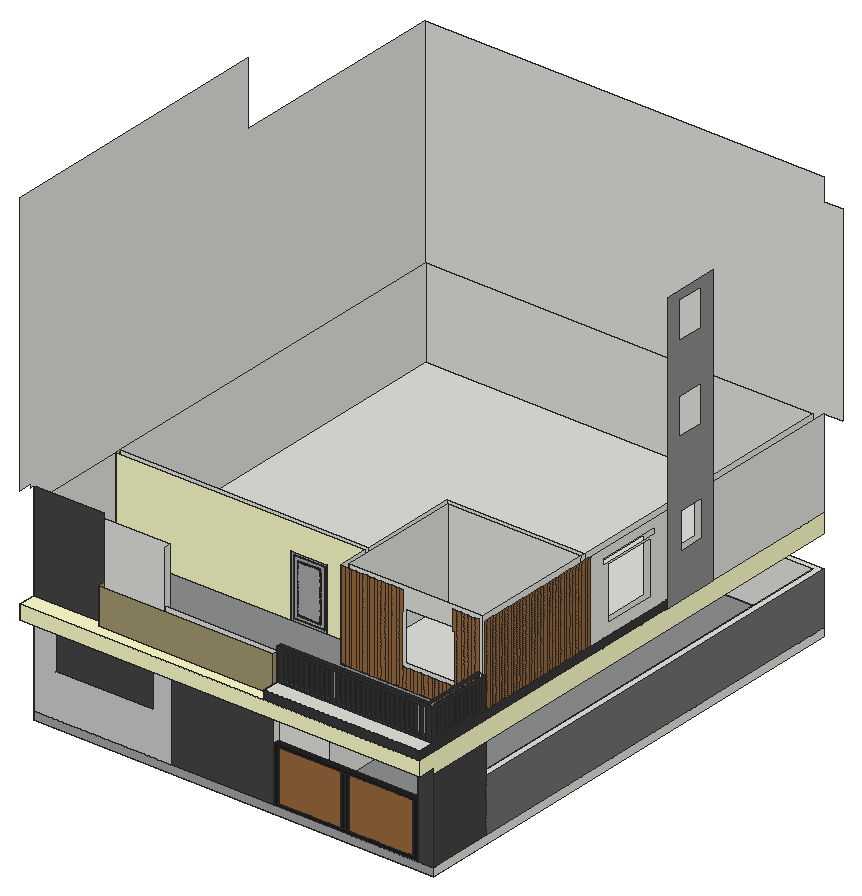
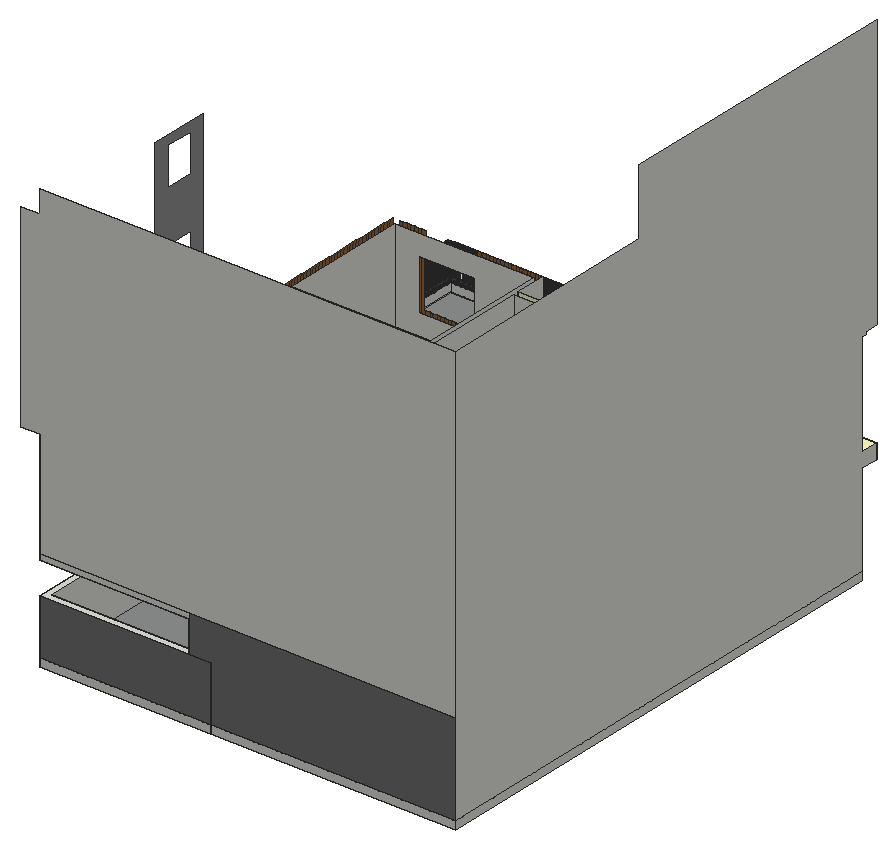
# SketchUp Ruby script. Lengths in inches.
U = 1.inch
M = Sketchup.active_model
def pt(a) = Geom::Point3d.new(a.map { |v| v * U })
def face(e, loops, mat)
  f = e.add_face(loops[0].map { |a| pt(a) })
  loops[1..].each { |l| e.add_face(l.map { |a| pt(a) }).erase! }
  f.material = f.back_material = mat if mat
  f
end
# faces: each face lists its corners as indices into pts; further lists are holes
def faces(e, pts, list, mat = nil) = list.each { |f| face(e, (f[0].is_a?(Array) ? f : [f]).map { |l| l.map { |i| pts[i] } }, mat) }
# xy, xz, yz: faces in a plane at the given z, y or x. An outline is a flat list of corners, or four numbers for a rectangle; further outlines are holes
def ring(l) = l.size == 4 ? [[l[0], l[1]], [l[2], l[1]], [l[2], l[3]], [l[0], l[3]]] : l.each_slice(2).to_a
def flat(e, list, mat, &to3) = list.each { |f| face(e, (f[0].is_a?(Array) ? f : [f]).map { |l| ring(l).map { |u, v| to3.(u, v) } }, mat) }
def xy(e, z, list, mat = nil) = flat(e, list, mat) { |x, y| [x, y, z] }
def xz(e, y, list, mat = nil) = flat(e, list, mat) { |x, z| [x, y, z] }
def yz(e, x, list, mat = nil) = flat(e, list, mat) { |y, z| [x, y, z] }
def lines(e, pts, list) = list.each { |a, b| e.add_line(pt(pts[a]), pt(pts[b])) }
# prism: a flat outline (further loops are holes) pulled along v
def prism(e, loops, v, mat = nil)
  f = face(e, loops, mat); d = Geom::Vector3d.new(v.map { |x| x * U })
  f.pushpull(f.normal.samedirection?(d) ? d.length : -d.length)
end
def box(e, o, s, mat = nil) = prism(e, [[o, [o[0] + s[0], o[1], o[2]], [o[0] + s[0], o[1] + s[1], o[2]], [o[0], o[1] + s[1], o[2]]]], [0, 0, s[2]], mat)
def at(x, y, z, deg = 0) = Geom::Transformation.translation(pt([x, y, z])) * Geom::Transformation.rotation(ORIGIN, Z_AXIS, deg.degrees)
def axes(o, x, y, z) = Geom::Transformation.new([*x, 0, *y, 0, *z, 0, *pt(o).to_a, 1])
def part(name) = M.definitions.add(name)
# library, detail: a bought-in or finely detailed component or shape, given as its bounding box
def library(name, o, s) = part(name).tap { |d| box(d.entities, o, s) }
def detail(e, o, s) = box(e.add_group.entities, o, s)
def put(e, d, t, mat = nil) = e.add_instance(d, t).tap { |i| i.material = mat if mat }
def group(e, t, mat = nil) = e.add_group.tap { |g| g.transformation = t; g.material = mat if mat }.entities
root = M.entities
M.materials.add("[Blacktop Old 02]").color = [143, 145, 145]
M.materials.add("[Carrera Marble]").color = [207, 207, 207]
M.materials.add("[Color A08]1").color = [91, 11, 0]
M.materials.add("[Color E01]").color = [255, 255, 204]
M.materials.add("[Color M03]").color = [170, 170, 170]
M.materials.add("[Color M04]").color = [142, 142, 142]
M.materials.add("[Color M05]").color = [114, 114, 114]
M.materials.add("[Color M07]").color = [58, 58, 58]
M.materials.add("[Color M08]").color = [30, 30, 30]
M.materials.add("[Granite Dark Gray]1").color = [69, 68, 68]
M.materials.add("[Granite Dark Gray]2").color = [69, 68, 68]
M.materials.add("[Stone Vein Gray]").color = [166, 165, 165]
M.materials.add("[Wood Floor]").color = [155, 105, 61]
M.materials.add("[Wood Lumber ButtJoined]").color = [164, 152, 112]
c1 = part("Group\#3")
xy(c1.entities,0,[[0,0,48,5]],"[Color M03]")
xy(c1.entities,2.98,[[2.98,0,45.02,5]],"[Color M03]")
xy(c1.entities,81.02,[[2.98,0,45.02,5]],"[Color M03]")
xy(c1.entities,84,[[0,0,48,5]],"[Color M03]")
xz(c1.entities,0,[[[2.98,2.98,45.02,81.02],[4.42,4.42,43.58,79.58]],[[8.55,8.55,39.45,75.45],[9.61,9.61,38.39,74.39]]],"[Color A08]1")
xz(c1.entities,0,[[[0,0,48,84],[2.98,2.98,45.02,81.02]],[[4.42,4.42,43.58,79.58],[8.55,8.55,39.45,75.45]],[9.61,9.61,38.39,74.39]],"[Color M03]")
xz(c1.entities,5,[[[0,0,48,84],[2.98,2.98,45.02,81.02]]],"[Color M03]")
yz(c1.entities,0,[[0,0,5,84]],"[Color M03]")
yz(c1.entities,2.98,[[0,2.98,5,81.02]],"[Color M03]")
yz(c1.entities,45.02,[[0,2.98,5,81.02]],"[Color M03]")
yz(c1.entities,48,[[0,0,5,84]],"[Color M03]")
xy(root,-10.6875,[[0,27,540,687]])
xy(root,0,[[[0,27,324.55,27,324.55,36,9,36,9,94.1875,345.75,94.1875,345.75,678,317.875,678,317.875,687,0,687],[9,100.1875,311.3125,678]],[324.55,27,518.875,36],[518.875,27,540,114.78],[9,100.1875,311.3125,678],[531,114.78,540,114.78,540,687,317.875,687,317.875,678,531,678]])
xy(root,0,[[9,36,518.875,36,518.875,114.78,531,114.78,531,678,345.75,678,345.75,94.1875,9,94.1875]],"[Blacktop Old 02]")
xy(root,72,[[531,114.78,540,114.78,540,687,345.75,687,345.75,678,531,678],[317.875,678,345.75,687]])
xy(root,102.125,[[9,100.1875,311.3125,678]])
xy(root,113.5625,[[324.55,27,324.55,94.1875,345.75,94.1875,345.75,687,531,687,531,114.78,518.875,114.78,518.875,27],[518.875,27,531,36],[518.875,36,531,114.78],[531,114.78,540,687]])
xy(root,116.6875,[[9,36,324.55,94.1875]])
xy(root,120,[[0,3.875,324.55,27],[324.55,3.875,531,27],[531,3.875,540,27]])
xy(root,139.5625,[[330.17,3.875,540,27],[176.76,27,176.76,31.22,531,31.22,531,113.4375,540,113.4375,540,27],[351.1875,121.0625,531,288],[9,161.0625,345.1875,161.0625,345.1875,294,531,294,531,678,9,678]])
xy(root,139.5625,[[0,3.875,330.17,3.875,330.17,18,94.8,18,94.8,27,0,27]],"[Color E01]")
xy(root,140.19,[[176.76,31.22,531,31.22,531,113.4375,345.1875,113.4375,345.1875,154.125,294.2,154.125,294.2,161.0625,246.2,161.0625,246.2,154.125,9,154.125,9,36,176.76,36]],"[Blacktop Old 02]")
xy(root,151.5625,[[330.17,3.875,540,24.875],[330.17,24.875,330.17,31.22,531,31.22,531,113.4375,540,113.4375,540,24.875],[176.76,27,330.17,31.22]])
xy(root,154.78,[[337.98,26.53,339.42,29.97],[344.98,26.53,346.42,29.97],[488.48,26.53,489.92,29.97],[494.98,26.53,496.42,29.97],[501.48,26.53,502.92,29.97],
  [507.98,26.53,509.42,29.97],[514.3,26.53,515.73,29.97],[522.48,26.53,523.92,29.97]])
xy(root,154.78,[[[333.39,24.875,531,31.22],[337.98,26.53,339.42,29.97],[344.98,26.53,346.42,29.97],[351.98,26.53,353.42,29.97],[358.98,26.53,360.42,29.97],[365.98,26.53,367.42,29.97],[372.98,26.53,374.42,29.97],[379.98,26.53,381.42,29.97],[386.98,26.53,388.42,29.97],[393.98,26.53,395.42,29.97],[400.98,26.53,402.42,29.97],[407.98,26.53,409.42,29.97],[414.98,26.53,416.42,29.97],[421.98,26.53,423.42,29.97],[428.98,26.53,430.42,29.97],[435.98,26.53,437.42,29.97],[442.98,26.53,444.42,29.97],[449.48,26.53,450.92,29.97],[455.98,26.53,457.42,29.97],[462.48,26.53,463.92,29.97],[468.98,26.53,470.42,29.97],[475.48,26.53,476.92,29.97],[481.98,26.53,483.42,29.97],[488.48,26.53,489.92,29.97],[494.98,26.53,496.42,29.97],[501.48,26.53,502.92,29.97],[507.98,26.53,509.42,29.97],[514.3,26.53,515.73,29.97],[522.48,26.53,523.92,29.97]]],"[Color M07]")
xy(root,155.78,[[533.85,35.98,537.54,37.92],[533.85,42.8,537.54,44.73],[533.85,49.61,537.54,51.55],[533.85,56.42,537.54,58.36],[533.85,63.23,537.54,65.17],
  [533.85,70.05,537.54,71.98],[533.85,76.86,537.54,78.8],[533.85,83.67,537.54,85.61],[533.85,90.48,537.54,92.42],[533.85,97.3,537.54,99.23],
  [533.85,104.11,537.54,106.05]])
xy(root,155.78,[[[531,31.22,540,109.22],[533.85,35.98,537.54,37.92],[533.85,42.8,537.54,44.73],[533.85,49.61,537.54,51.55],[533.85,56.42,537.54,58.36],[533.85,63.23,537.54,65.17],[533.85,70.05,537.54,71.98],[533.85,76.86,537.54,78.8],[533.85,83.67,537.54,85.61],[533.85,90.48,537.54,92.42],[533.85,97.3,537.54,99.23],[533.85,104.11,537.54,106.05]]],"[Color M07]")
xz(root,3.875,[[0,120,540,139.5625]],"[Color E01]")
xz(root,3.875,[[330.17,139.5625,540,151.5625]],"[Color M07]")
xz(root,18,[[94.8,139.5625,330.17,188.5625]],"[Wood Lumber ButtJoined]")
xz(root,24.875,[[330.17,151.5625,531,151.5625,531,154.78,333.39,154.78,333.39,192.35,531,192.35,531,195.5625,330.17,195.5625],[531,151.5625,540,195.5625]],"[Color M07]")
xz(root,26.53,[[337.98,154.78,339.42,192.35],[344.98,154.78,346.42,192.09],[351.98,154.78,353.42,192.4],[358.98,154.78,360.42,192.35],[365.98,154.78,367.42,192.34],
  [372.98,154.78,374.42,192.28],[379.98,154.78,381.42,192.65],[386.98,154.78,388.42,193.16],[393.98,154.78,395.42,192.35],[400.98,154.78,402.42,192.35],
  [407.98,154.78,409.42,192.35],[414.98,154.78,416.42,193.4],[421.98,154.78,423.42,193.03],[428.98,154.78,430.42,192.35],[435.98,154.78,437.42,192.4],
  [442.98,154.78,444.42,193.47],[449.48,154.78,450.92,192.35],[455.98,154.78,457.42,192.28],[462.48,154.78,463.92,194.84],[468.98,154.78,470.42,192.34],
  [475.48,154.78,476.92,192.35],[481.98,154.78,483.42,192.34],[488.48,154.78,489.92,192.35],[494.98,154.78,496.42,192.35],[501.48,154.78,502.92,192.34],
  [507.98,154.78,509.42,192.35],[514.3,154.78,515.73,192.35],[522.48,154.78,523.92,195.5625]],"[Color M07]")
xz(root,27,[[176.76,139.5625,330.17,151.5625],[176.76,151.5625,330.17,188.5625]])
xz(root,27,[[[0,0,184.8,120],[29.8,57.58,161.98,104.58]]],"[Carrera Marble]")
xz(root,27,[[184.8,0,324.55,0,324.55,113.5625,531,113.5625,531,120,184.8,120],[0,139.5625,94.8,272.3125]],"[Granite Dark Gray]1")
xz(root,27,[[518.875,0,540,0,540,120,531,120,531,113.5625,518.875,113.5625],[29.8,57.58,161.98,104.58]],"[Granite Dark Gray]2")
xz(root,27,[[0,-10.6875,540,0]],"[Stone Vein Gray]")
xz(root,29.97,[[337.98,154.78,339.42,192.35],[344.98,154.78,346.42,192.09],[351.98,154.78,353.42,192.4],[358.98,154.78,360.42,192.35],[365.98,154.78,367.42,192.34],
  [372.98,154.78,374.42,192.28],[379.98,154.78,381.42,192.65],[386.98,154.78,388.42,193.16],[393.98,154.78,395.42,192.35],[400.98,154.78,402.42,192.35],
  [407.98,154.78,409.42,192.35],[414.98,154.78,416.42,193.4],[421.98,154.78,423.42,193.03],[428.98,154.78,430.42,192.35],[435.98,154.78,437.42,192.4],
  [442.98,154.78,444.42,193.47],[449.48,154.78,450.92,192.35],[455.98,154.78,457.42,192.28],[462.48,154.78,463.92,194.84],[468.98,154.78,470.42,192.34],
  [475.48,154.78,476.92,192.35],[481.98,154.78,483.42,192.34],[488.48,154.78,489.92,192.35],[494.98,154.78,496.42,192.35],[501.48,154.78,502.92,192.34],
  [507.98,154.78,509.42,192.35],[514.3,154.78,515.73,192.35],[522.48,154.78,523.92,195.5625]],"[Color M07]")
xz(root,31.22,[[176.76,139.5625,531,140.19],[176.76,140.19,531,151.5625]])
xz(root,31.22,[[330.17,151.5625,330.17,195.5625,531,195.5625,531,192.35,333.39,192.35,333.39,154.78,531,154.78,531,151.5625],[531,155.78,540,191.35]],"[Color M07]")
xz(root,35.98,[[533.85,155.78,537.54,191.28]],"[Color M07]")
xz(root,36,[[9,0,324.55,116.6875],[9,139.5625,176.76,140.19],[9,140.19,176.76,259.5625]])
xz(root,37.92,[[533.85,155.78,537.54,191.28]],"[Color M07]")
xz(root,42.8,[[533.85,155.78,537.54,191.4]],"[Color M07]")
xz(root,44.73,[[533.85,155.78,537.54,191.4]],"[Color M07]")
xz(root,49.61,[[533.85,155.78,537.54,191.34]],"[Color M07]")
xz(root,51.55,[[533.85,155.78,537.54,191.34]],"[Color M07]")
xz(root,56.42,[[533.85,155.78,537.54,191.35]],"[Color M07]")
xz(root,58.36,[[533.85,155.78,537.54,191.35]],"[Color M07]")
xz(root,63.23,[[533.85,155.78,537.54,191.53]],"[Color M07]")
xz(root,65.17,[[533.85,155.78,537.54,191.53]],"[Color M07]")
xz(root,70.05,[[533.85,155.78,537.54,191.47]],"[Color M07]")
xz(root,71.98,[[533.85,155.78,537.54,191.47]],"[Color M07]")
xz(root,76.86,[[533.85,155.78,537.54,191.53]],"[Color M07]")
xz(root,78.8,[[533.85,155.78,537.54,191.53]],"[Color M07]")
xz(root,83.67,[[533.85,155.78,537.54,191.35]],"[Color M07]")
xz(root,85.61,[[533.85,155.78,537.54,191.35]],"[Color M07]")
xz(root,90.48,[[533.85,155.78,537.54,191.35]],"[Color M07]")
xz(root,92.42,[[533.85,155.78,537.54,191.35]],"[Color M07]")
xz(root,94.1875,[[9,0,345.75,0,345.75,113.5625,324.55,113.5625,324.55,116.6875,9,116.6875]])
xz(root,97.3,[[533.85,155.78,537.54,191.34]],"[Color M07]")
xz(root,99.23,[[533.85,155.78,537.54,191.34]],"[Color M07]")
xz(root,100.1875,[[9,0,311.3125,102.125]])
xz(root,104.11,[[533.85,155.78,537.54,191.78]],"[Color M07]")
xz(root,106.05,[[533.85,155.78,537.54,191.78]],"[Color M07]")
xz(root,109.22,[[531,155.78,540,191.35]],"[Color M07]")
xz(root,113.4375,[[345.1875,139.5625,531,140.19],[531,151.5625,531.62,195.5625],[531.62,151.5625,536.49,195.5625],[536.49,151.5625,540,195.5625]])
xz(root,113.4375,[[345.1875,140.19,351.24,259.5625],[351.24,140.19,356.12,259.5625],[356.12,140.19,360.99,259.5625],[360.99,140.19,365.87,259.5625],[365.87,140.19,370.74,259.5625],
  [370.74,140.19,375.62,259.5625],[375.62,140.19,380.49,259.5625],[380.49,140.19,385.37,259.5625],[385.37,140.19,390.24,259.5625],[390.24,140.19,395.12,259.5625],
  [395.12,140.19,399.99,259.5625],[399.99,140.19,404.87,259.5625],[404.87,140.19,409.74,259.5625],[409.74,140.19,414.62,259.5625],[414.62,140.19,419.49,259.5625],
  [419.49,140.19,424.37,259.5625],[424.37,140.19,429.24,140.19,429.24,166.65,427.93,166.65,427.93,232.9,429.24,232.9,429.24,259.5625,424.37,259.5625],[429.24,140.19,434.12,166.65],[434.12,140.19,438.99,166.65],[438.99,140.19,443.87,166.65],
  [443.87,140.19,448.74,166.65],[448.74,140.19,453.62,166.65],[453.62,140.19,458.49,166.65],[458.49,140.19,463.37,166.65],[463.37,140.19,468.24,166.65],
  [468.24,140.19,473.12,166.65],[473.12,140.19,477.99,166.65],[477.99,140.19,482.87,166.65],[482.87,140.19,487.74,166.65],[487.74,140.19,492.62,166.65],
  [492.62,140.19,497.49,166.65],[497.49,140.19,502.37,140.19,502.37,259.5625,497.49,259.5625,497.49,232.9,499.81,232.9,499.81,166.65,497.49,166.65],[502.37,140.19,507.24,259.5625],[507.24,140.19,512.12,259.5625],[512.12,140.19,516.99,259.5625],
  [516.99,140.19,521.87,259.5625],[521.87,140.19,526.74,259.5625],[526.74,140.19,531,140.19,531,195.5625,531.62,195.5625,531.62,259.5625,526.74,259.5625]],"[Wood Floor]")
xz(root,114.78,[[518.875,0,531,72],[531,0,540,72]])
xz(root,114.78,[[518.875,72,540,113.5625]],"[Granite Dark Gray]2")
xz(root,121.0625,[[[351.1875,139.5625,531,259.5625],[427.93,166.65,499.81,232.9]]])
xz(root,154.125,[[9,140.19,246.2,140.19,246.2,224.19,294.2,224.19,294.2,140.19,345.1875,140.19,345.1875,259.5625,9,259.5625]],"[Color E01]")
xz(root,161.0625,[[[9,139.5625,345.1875,259.5625],[246.2,140.19,294.2,224.19]]])
xz(root,288,[[351.1875,139.5625,531,259.5625]])
xz(root,294,[[345.1875,139.5625,531,259.5625]])
xz(root,678,[[9,-10.6875,311.3125,0],[317.875,-10.6875,531,0],[9,0,311.3125,102.125],[317.875,0,345.75,72],[345.75,0,531,72],
  [9,139.5625,345.75,259.5625],[345.75,139.5625,531,259.5625]])
xz(root,687,[[0,-10.6875,317.875,0],[317.875,-10.6875,540,0],[345.75,113.5625,540,120],[0,120,0,545.5625,540,545.5625,540,515.86,564.9375,515.86,564.9375,259.5625,540,259.5625,540,120]])
xz(root,687,[[0,0,0,120,345.75,120,345.75,72,317.875,72,317.875,0],[317.875,0,540,72]],"[Color M05]")
yz(root,0,[[27,-10.6875,687,0],[27,0,27,120,3.875,120,3.875,139.5625,27,139.5625,27,272.3125,21.625,272.3125,21.625,276.5625,3.875,276.5625,3.875,631.3125,388.6875,631.3125,388.6875,545.5625,687,545.5625,687,0]])
yz(root,9,[[36,0,94.1875,116.6875],[100.1875,0,678,102.125],[36,139.5625,113.4375,140.19],[113.4375,139.5625,161.0625,139.5625,161.0625,259.5625,154.125,259.5625,154.125,140.19,113.4375,140.19],[161.0625,139.5625,678,259.5625],
  [36,140.19,154.125,259.5625]])
yz(root,94.8,[[18,139.5625,27,188.5625]],"[Wood Lumber ButtJoined]")
yz(root,176.76,[[27,139.5625,31.22,151.5625],[31.22,139.5625,36,140.19],[31.22,140.19,36,151.5625],[27,151.5625,36,259.5625]])
yz(root,246.2,[[154.125,140.19,161.0625,224.19]])
yz(root,294.2,[[154.125,140.19,161.0625,224.19]])
yz(root,311.3125,[[100.1875,0,678,102.125]])
yz(root,317.875,[[678,-10.6875,687,0],[678,0,687,72]])
yz(root,324.55,[[27,0,36,113.5625]])
yz(root,330.17,[[3.875,139.5625,18,151.5625],[18,139.5625,27,151.5625],[24.875,151.5625,27,188.5625]])
yz(root,330.17,[[27,151.5625,27,188.5625,24.875,188.5625,24.875,195.5625,31.22,195.5625,31.22,151.5625]],"[Color M07]")
yz(root,330.17,[[18,151.5625,24.875,188.5625]],"[Wood Lumber ButtJoined]")
yz(root,333.39,[[24.875,154.78,31.22,188.5625]],"[Color M07]")
yz(root,337.98,[[26.53,154.78,29.97,192.35]],"[Color M07]")
yz(root,339.42,[[26.53,154.78,29.97,192.35]],"[Color M07]")
yz(root,344.98,[[26.53,154.78,29.97,192.09]],"[Color M07]")
yz(root,345.1875,[[161.0625,139.5625,294,259.5625],[113.4375,140.19,154.125,259.5625]])
yz(root,345.75,[[94.1875,0,678,0,678,72,687,72,687,113.5625,94.1875,113.5625]])
yz(root,346.42,[[26.53,154.78,29.97,192.09]],"[Color M07]")
yz(root,351.1875,[[121.0625,139.5625,288,259.5625]])
yz(root,351.98,[[26.53,154.78,29.97,192.4]],"[Color M07]")
yz(root,353.42,[[26.53,154.78,29.97,192.4]],"[Color M07]")
yz(root,358.98,[[26.53,154.78,29.97,192.35]],"[Color M07]")
yz(root,360.42,[[26.53,154.78,29.97,192.35]],"[Color M07]")
yz(root,365.98,[[26.53,154.78,29.97,192.34]],"[Color M07]")
yz(root,367.42,[[26.53,154.78,29.97,192.34]],"[Color M07]")
yz(root,372.98,[[26.53,154.78,29.97,192.28]],"[Color M07]")
yz(root,374.42,[[26.53,154.78,29.97,192.28]],"[Color M07]")
yz(root,379.98,[[26.53,154.78,29.97,192.65]],"[Color M07]")
yz(root,381.42,[[26.53,154.78,29.97,192.65]],"[Color M07]")
yz(root,386.98,[[26.53,154.78,29.97,193.16]],"[Color M07]")
yz(root,388.42,[[26.53,154.78,29.97,193.16]],"[Color M07]")
yz(root,393.98,[[26.53,154.78,29.97,192.35]],"[Color M07]")
yz(root,395.42,[[26.53,154.78,29.97,192.35]],"[Color M07]")
yz(root,400.98,[[26.53,154.78,29.97,192.35]],"[Color M07]")
yz(root,402.42,[[26.53,154.78,29.97,192.35]],"[Color M07]")
yz(root,407.98,[[26.53,154.78,29.97,192.35]],"[Color M07]")
yz(root,409.42,[[26.53,154.78,29.97,192.35]],"[Color M07]")
yz(root,414.98,[[26.53,154.78,29.97,193.4]],"[Color M07]")
yz(root,416.42,[[26.53,154.78,29.97,193.4]],"[Color M07]")
yz(root,421.98,[[26.53,154.78,29.97,193.03]],"[Color M07]")
yz(root,423.42,[[26.53,154.78,29.97,193.03]],"[Color M07]")
yz(root,428.98,[[26.53,154.78,29.97,192.35]],"[Color M07]")
yz(root,430.42,[[26.53,154.78,29.97,192.35]],"[Color M07]")
yz(root,435.98,[[26.53,154.78,29.97,192.4]],"[Color M07]")
yz(root,437.42,[[26.53,154.78,29.97,192.4]],"[Color M07]")
yz(root,442.98,[[26.53,154.78,29.97,193.47]],"[Color M07]")
yz(root,444.42,[[26.53,154.78,29.97,193.47]],"[Color M07]")
yz(root,449.48,[[26.53,154.78,29.97,192.35]],"[Color M07]")
yz(root,450.92,[[26.53,154.78,29.97,192.35]],"[Color M07]")
yz(root,455.98,[[26.53,154.78,29.97,192.28]],"[Color M07]")
yz(root,457.42,[[26.53,154.78,29.97,192.28]],"[Color M07]")
yz(root,462.48,[[26.53,154.78,29.97,194.84]],"[Color M07]")
yz(root,463.92,[[26.53,154.78,29.97,194.84]],"[Color M07]")
yz(root,468.98,[[26.53,154.78,29.97,192.34]],"[Color M07]")
yz(root,470.42,[[26.53,154.78,29.97,192.34]],"[Color M07]")
yz(root,475.48,[[26.53,154.78,29.97,192.35]],"[Color M07]")
yz(root,476.92,[[26.53,154.78,29.97,192.35]],"[Color M07]")
yz(root,481.98,[[26.53,154.78,29.97,192.34]],"[Color M07]")
yz(root,483.42,[[26.53,154.78,29.97,192.34]],"[Color M07]")
yz(root,488.48,[[26.53,154.78,29.97,192.35]],"[Color M07]")
yz(root,489.92,[[26.53,154.78,29.97,192.35]],"[Color M07]")
yz(root,494.98,[[26.53,154.78,29.97,192.35]],"[Color M07]")
yz(root,496.42,[[26.53,154.78,29.97,192.35]],"[Color M07]")
yz(root,501.48,[[26.53,154.78,29.97,192.34]],"[Color M07]")
yz(root,502.92,[[26.53,154.78,29.97,192.34]],"[Color M07]")
yz(root,507.98,[[26.53,154.78,29.97,192.35]],"[Color M07]")
yz(root,509.42,[[26.53,154.78,29.97,192.35]],"[Color M07]")
yz(root,514.3,[[26.53,154.78,29.97,192.35]],"[Color M07]")
yz(root,515.73,[[26.53,154.78,29.97,192.35]],"[Color M07]")
yz(root,518.875,[[27,0,36,113.5625],[36,0,114.78,113.5625]],"[Granite Dark Gray]2")
yz(root,522.48,[[26.53,154.78,29.97,195.5625]],"[Color M07]")
yz(root,523.92,[[26.53,154.78,29.97,195.5625]],"[Color M07]")
yz(root,531,[[114.78,0,678,72],[27,113.5625,114.78,120],[31.22,139.5625,113.4375,140.19],[121.0625,139.5625,288,259.5625],[288,139.5625,294,259.5625],
  [[294,139.5625,678,259.5625],[322.23,166.03,393.92,237.71],[443.95,199.38,480.39,248.63]],[31.22,140.19,113.4375,151.5625]])
yz(root,531,[[31.22,151.5625,31.22,155.78,109.22,155.78,109.22,191.35,31.22,191.35,31.22,195.5625,113.4375,195.5625,113.4375,151.5625],[24.875,154.78,31.22,192.35]],"[Color M07]")
yz(root,533.85,[[35.98,155.78,37.92,191.28],[42.8,155.78,44.73,191.4],[49.61,155.78,51.55,191.34],[56.42,155.78,58.36,191.35],[63.23,155.78,65.17,191.53],
  [70.05,155.78,71.98,191.47],[76.86,155.78,78.8,191.53],[83.67,155.78,85.61,191.35],[90.48,155.78,92.42,191.35],[97.3,155.78,99.23,191.34],
  [104.11,155.78,106.05,191.78]],"[Color M07]")
yz(root,537.54,[[35.98,155.78,37.92,191.28],[42.8,155.78,44.73,191.4],[49.61,155.78,51.55,191.34],[56.42,155.78,58.36,191.35],[63.23,155.78,65.17,191.53],
  [70.05,155.78,71.98,191.47],[76.86,155.78,78.8,191.53],[83.67,155.78,85.61,191.35],[90.48,155.78,92.42,191.35],[97.3,155.78,99.23,191.34],
  [104.11,155.78,106.05,191.78]],"[Color M07]")
yz(root,540,[[27,-10.6875,687,0],[499.48,139.5625,687,259.5625],[[292.98,151.5625,421.98,259.5625],[322.23,166.03,393.92,237.71],[313.39,239.1,401.58,247.29]]])
yz(root,540,[[27,113.5625,687,113.5625,687,139.5625,3.875,139.5625,3.875,120,27,120]],"[Color E01]")
yz(root,540,[[[421.98,139.5625,499.48,515.86],[441.39,338.69,477.83,387.94],[441.79,455.03,478.23,504.28],[443.95,199.38,480.39,248.63]]],"[Color M04]")
yz(root,540,[[114.78,0,687,72]],"[Color M05]")
yz(root,540,[[3.875,139.5625,421.98,151.5625],[[24.875,151.5625,113.4375,195.5625],[31.22,155.78,109.22,191.35]]],"[Color M07]")
yz(root,540,[[27,0,114.78,113.5625]],"[Granite Dark Gray]2")
yz(root,540,[[113.4375,151.5625,117.98,259.5625],[117.98,151.5625,122.98,259.5625],[122.98,151.5625,127.98,259.5625],[127.98,151.5625,132.98,259.5625],[132.98,151.5625,137.98,259.5625],
  [137.98,151.5625,142.98,259.5625],[142.98,151.5625,147.98,259.5625],[147.98,151.5625,152.98,259.5625],[152.98,151.5625,157.98,259.5625],[157.98,151.5625,162.98,259.5625],
  [162.98,151.5625,167.98,259.5625],[167.98,151.5625,172.98,259.5625],[172.98,151.5625,177.98,259.5625],[177.98,151.5625,182.98,259.5625],[182.98,151.5625,187.98,259.5625],
  [187.98,151.5625,192.98,259.5625],[192.98,151.5625,197.98,259.5625],[197.98,151.5625,202.98,259.5625],[202.98,151.5625,207.98,259.5625],[207.98,151.5625,212.98,259.5625],
  [212.98,151.5625,217.98,259.5625],[217.98,151.5625,222.98,259.5625],[222.98,151.5625,227.98,259.5625],[227.98,151.5625,232.98,259.5625],[232.98,151.5625,237.98,259.5625],
  [237.98,151.5625,242.98,259.5625],[242.98,151.5625,247.98,259.5625],[247.98,151.5625,252.98,259.5625],[252.98,151.5625,257.98,259.5625],[257.98,151.5625,262.98,259.5625],
  [262.98,151.5625,267.98,259.5625],[267.98,151.5625,272.98,259.5625],[272.98,151.5625,277.98,259.5625],[277.98,151.5625,282.98,259.5625],[282.98,151.5625,287.98,259.5625],
  [287.98,151.5625,292.98,259.5625]],"[Wood Floor]")
p = [[9,94.1875,0],[9,94.1875,-10.6875],[317.875,94.1875,0],[317.875,94.1875,-10.6875],[9,36,0],[9,36,-10.6875],
  [9,100.1875,0],[9,100.1875,-10.6875],[311.3125,100.1875,0],[311.3125,100.1875,-10.6875],[531,36,0],[531,36,-10.6875],
  [531,114.78,120],[531,687,120],[345.75,94.1875,113.5625],[345.75,94.1875,120],[28,100.1875,120],[28,100.1875,102.125],
  [311.3125,678,102.125],[311.3125,678,120],[9,678,102.125],[9,678,120],[311.3125,100.1875,102.125],[311.3125,100.1875,120],
  [45.8125,36,120],[45.8125,36,116.6875],[9,36,116.6875],[9,36,120],[324.55,36,116.6875],[324.55,36,120],
  [324.55,27,120],[324.55,94.1875,116.6875],[324.55,94.1875,120],[540,114.78,120],[531,113.4375,139.5625],[531,121.0625,139.5625],
  [531.62,113.4375,151.5625],[531.62,113.4375,140.19],[536.49,113.4375,151.5625],[536.49,113.4375,140.19],[9,100.1875,102.125],[9,100.1875,120]]
lines(root,p,[[0,1],[2,3],[4,5],[6,7],[8,9],[10,11],[12,13],[14,15],[16,17],[18,19],[20,21],[22,23],
  [24,25],[26,27],[28,29],[29,30],[31,32],[12,33],[34,35],[36,37],[38,39],[40,41]])
g1 = group(root,at(324.55,27,0))
xy(g1,0,[[0,0,194.32,5]],"[Color M08]")
xy(g1,4.37,[[6.89,0,90.78,5],[90.78,0,96.28,5],[96.28,0,101.78,5],[101.78,0,187.43,5]],"[Color M08]")
xy(g1,71.73,[[6.89,0,90.78,5],[90.78,0,96.28,5],[96.28,0,101.78,5],[101.78,0,187.43,5]],"[Color M08]")
xy(g1,76.1,[[0,0,194.32,5]],"[Color M08]")
xz(g1,0,[[[0,0,194.32,76.1],[6.89,4.37,187.43,71.73]],[90.78,4.37,96.28,71.73],[96.28,4.37,101.78,71.73]],"[Color M08]")
xz(g1,0,[[6.89,4.37,90.78,71.73],[101.78,4.37,187.43,71.73]],"[Wood Floor]")
xz(g1,5,[[[0,0,194.32,76.1],[6.89,4.37,187.43,71.73]],[90.78,4.37,96.28,71.73],[96.28,4.37,101.78,71.73]],"[Color M08]")
xz(g1,5,[[6.89,4.37,90.78,71.73],[101.78,4.37,187.43,71.73]],"[Wood Floor]")
yz(g1,0,[[0,0,5,76.1]],"[Color M08]")
yz(g1,6.89,[[0,4.37,5,71.73]],"[Color M08]")
yz(g1,90.78,[[0,4.37,5,71.73]])
yz(g1,96.28,[[0,4.37,5,71.73]],"[Color M08]")
yz(g1,101.78,[[0,4.37,5,71.73]])
yz(g1,187.43,[[0,4.37,5,71.73]],"[Color M08]")
yz(g1,194.32,[[0,0,5,76.1]],"[Color M08]")
put(root,c1,at(246.2,154.125,140.19))
